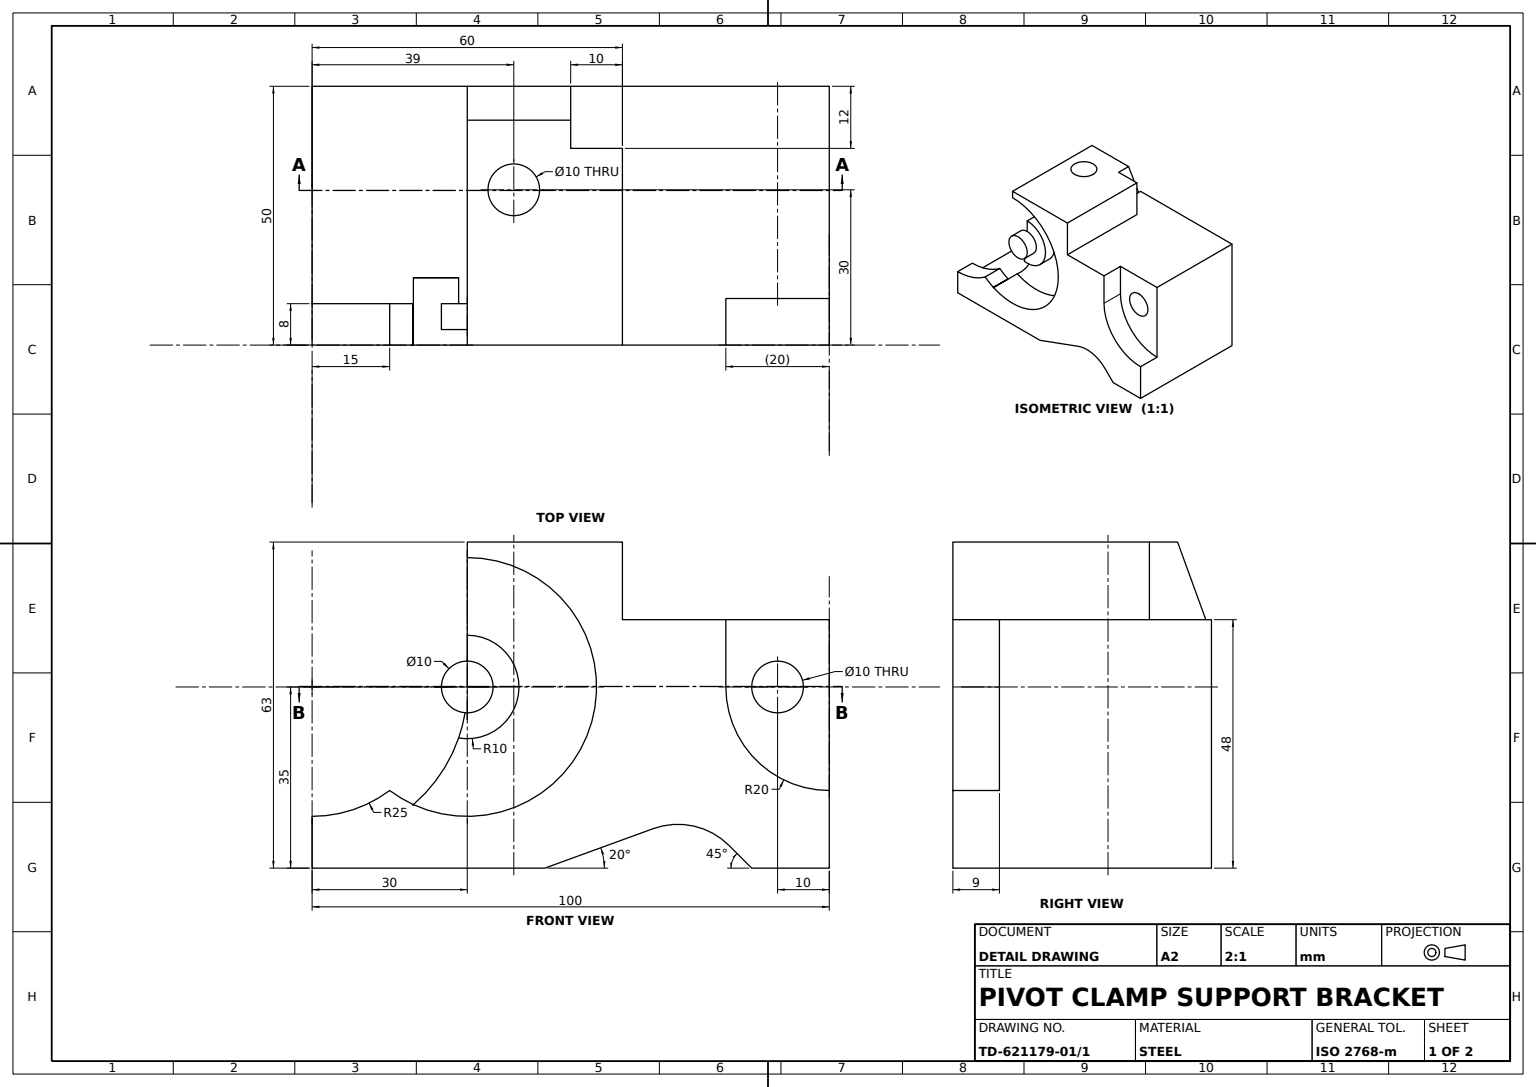
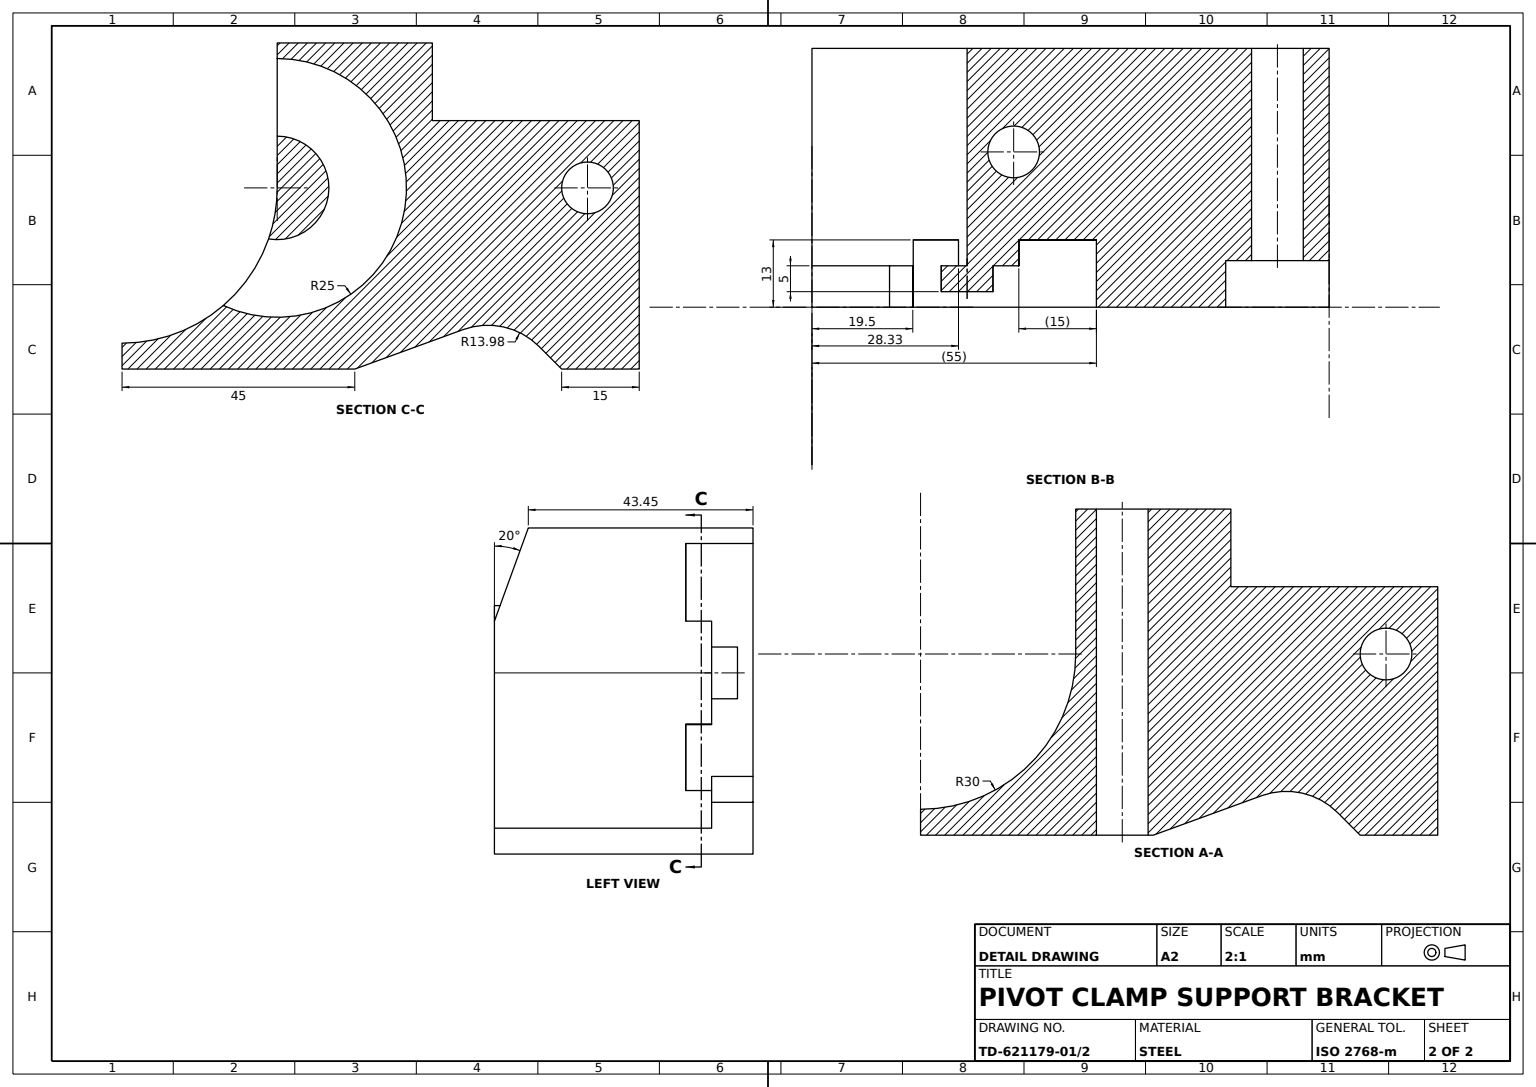
ISO-10303-21;
HEADER;
FILE_DESCRIPTION((''),'2;1');
FILE_NAME('','',(''),(''),'','','');
FILE_SCHEMA(('AUTOMOTIVE_DESIGN'));
ENDSEC;
DATA;
#1=APPLICATION_CONTEXT('');
#2=PRODUCT_CONTEXT('',#1,'mechanical');
#3=PRODUCT('','','',(#2));
#4=PRODUCT_DEFINITION_FORMATION('','',#3);
#5=PRODUCT_DEFINITION_CONTEXT('',#1,'design');
#6=PRODUCT_DEFINITION('','',#4,#5);
#7=PRODUCT_DEFINITION_SHAPE('','',#6);
#8=(LENGTH_UNIT()NAMED_UNIT(*)SI_UNIT(.MILLI.,.METRE.));
#9=(NAMED_UNIT(*)PLANE_ANGLE_UNIT()SI_UNIT($,.RADIAN.));
#10=(NAMED_UNIT(*)SI_UNIT($,.STERADIAN.)SOLID_ANGLE_UNIT());
#11=UNCERTAINTY_MEASURE_WITH_UNIT(LENGTH_MEASURE(0.005),#8,'distance_accuracy_value','');
#12=(GEOMETRIC_REPRESENTATION_CONTEXT(3)GLOBAL_UNCERTAINTY_ASSIGNED_CONTEXT((#11))GLOBAL_UNIT_ASSIGNED_CONTEXT((#8,#9,#10))REPRESENTATION_CONTEXT('',''));
#13=CARTESIAN_POINT('',(-25.,20.954127,-23.873322));
#14=VERTEX_POINT('',#13);
#15=CARTESIAN_POINT('',(25.,20.954127,-23.873322));
#16=VERTEX_POINT('',#15);
#17=CARTESIAN_POINT('',(48.,20.954127,-23.873322));
#18=DIRECTION('',(-1.,0.,0.));
#19=VECTOR('',#18,1000.);
#20=LINE('',#17,#19);
#21=EDGE_CURVE('',#14,#16,#20,.F.);
#22=ORIENTED_EDGE('',*,*,#21,.F.);
#23=CARTESIAN_POINT('',(-25.,35.625997,-27.125997));
#24=VERTEX_POINT('',#23);
#25=CARTESIAN_POINT('',(-25.,25.737223,-37.014771));
#26=DIRECTION('',(1.,0.,0.));
#27=DIRECTION('',(0.,0.,-1.));
#28=AXIS2_PLACEMENT_3D('',#25,#26,#27);
#29=CIRCLE('',#28,13.984838);
#30=EDGE_CURVE('',#24,#14,#29,.T.);
#31=ORIENTED_EDGE('',*,*,#30,.F.);
#32=CARTESIAN_POINT('',(25.,35.625997,-27.125997));
#33=VERTEX_POINT('',#32);
#34=CARTESIAN_POINT('',(48.,35.625997,-27.125997));
#35=LINE('',#34,#19);
#36=EDGE_CURVE('',#24,#33,#35,.F.);
#37=ORIENTED_EDGE('',*,*,#36,.T.);
#38=CARTESIAN_POINT('',(25.,25.737223,-37.014771));
#39=AXIS2_PLACEMENT_3D('',#38,#26,#27);
#40=CIRCLE('',#39,13.984838);
#41=EDGE_CURVE('',#33,#16,#40,.T.);
#42=ORIENTED_EDGE('',*,*,#41,.T.);
#43=EDGE_LOOP('',(#22,#31,#37,#42));
#44=FACE_BOUND('',#43,.T.);
#45=CARTESIAN_POINT('',(48.,25.737223,-37.014771));
#46=DIRECTION('',(0.,0.,1.));
#47=AXIS2_PLACEMENT_3D('',#45,#18,#46);
#48=CYLINDRICAL_SURFACE('',#47,13.984838);
#49=ADVANCED_FACE('',(#44),#48,.F.);
#50=CARTESIAN_POINT('',(17.,-25.5,-19.188103));
#51=VERTEX_POINT('',#50);
#52=CARTESIAN_POINT('',(17.,-30.,-16.5));
#53=VERTEX_POINT('',#52);
#54=CARTESIAN_POINT('',(17.,-15.,3.5));
#55=AXIS2_PLACEMENT_3D('',#54,#26,#27);
#56=CIRCLE('',#55,25.);
#57=EDGE_CURVE('',#51,#53,#56,.F.);
#58=ORIENTED_EDGE('',*,*,#57,.T.);
#59=CARTESIAN_POINT('',(25.,-30.,-16.5));
#60=VERTEX_POINT('',#59);
#61=CARTESIAN_POINT('',(27.5,-30.,-16.5));
#62=LINE('',#61,#19);
#63=EDGE_CURVE('',#60,#53,#62,.T.);
#64=ORIENTED_EDGE('',*,*,#63,.F.);
#65=CARTESIAN_POINT('',(25.,-25.5,-19.188103));
#66=VERTEX_POINT('',#65);
#67=CARTESIAN_POINT('',(25.,-15.,3.5));
#68=AXIS2_PLACEMENT_3D('',#67,#26,#27);
#69=CIRCLE('',#68,25.);
#70=EDGE_CURVE('',#66,#60,#69,.F.);
#71=ORIENTED_EDGE('',*,*,#70,.F.);
#72=CARTESIAN_POINT('',(49.,-25.5,-19.188103));
#73=LINE('',#72,#19);
#74=EDGE_CURVE('',#66,#51,#73,.T.);
#75=ORIENTED_EDGE('',*,*,#74,.T.);
#76=EDGE_LOOP('',(#58,#64,#71,#75));
#77=FACE_BOUND('',#76,.T.);
#78=CARTESIAN_POINT('',(49.,-15.,3.5));
#79=AXIS2_PLACEMENT_3D('',#78,#18,#46);
#80=CYLINDRICAL_SURFACE('',#79,25.);
#81=ADVANCED_FACE('',(#77),#80,.F.);
#82=CARTESIAN_POINT('',(17.,-45.,-21.5));
#83=VERTEX_POINT('',#82);
#84=CARTESIAN_POINT('',(17.,-45.,-26.5));
#85=VERTEX_POINT('',#84);
#86=CARTESIAN_POINT('',(17.,-45.,-16.276455));
#87=VECTOR('',#27,1000.);
#88=LINE('',#86,#87);
#89=EDGE_CURVE('',#83,#85,#88,.T.);
#90=ORIENTED_EDGE('',*,*,#89,.T.);
#91=CARTESIAN_POINT('',(-25.,-45.,-26.5));
#92=VERTEX_POINT('',#91);
#93=CARTESIAN_POINT('',(44.,-45.,-26.5));
#94=LINE('',#93,#19);
#95=EDGE_CURVE('',#92,#85,#94,.F.);
#96=ORIENTED_EDGE('',*,*,#95,.F.);
#97=CARTESIAN_POINT('',(-25.,-45.,-31.5));
#98=VERTEX_POINT('',#97);
#99=CARTESIAN_POINT('',(-25.,-45.,31.5));
#100=LINE('',#99,#87);
#101=EDGE_CURVE('',#92,#98,#100,.T.);
#102=ORIENTED_EDGE('',*,*,#101,.T.);
#103=CARTESIAN_POINT('',(25.,-45.,-31.5));
#104=VERTEX_POINT('',#103);
#105=LINE('',#103,#19);
#106=EDGE_CURVE('',#104,#98,#105,.T.);
#107=ORIENTED_EDGE('',*,*,#106,.F.);
#108=CARTESIAN_POINT('',(25.,-45.,-21.5));
#109=VERTEX_POINT('',#108);
#110=CARTESIAN_POINT('',(25.,-45.,31.5));
#111=LINE('',#110,#87);
#112=EDGE_CURVE('',#109,#104,#111,.T.);
#113=ORIENTED_EDGE('',*,*,#112,.F.);
#114=CARTESIAN_POINT('',(28.,-45.,-21.5));
#115=LINE('',#114,#19);
#116=EDGE_CURVE('',#83,#109,#115,.F.);
#117=ORIENTED_EDGE('',*,*,#116,.F.);
#118=EDGE_LOOP('',(#90,#96,#102,#107,#113,#117));
#119=FACE_BOUND('',#118,.T.);
#120=DIRECTION('',(0.,1.,0.));
#121=AXIS2_PLACEMENT_3D('',#110,#120,#46);
#122=PLANE('',#121);
#123=ADVANCED_FACE('',(#119),#122,.F.);
#124=CARTESIAN_POINT('',(22.,-10.,3.5));
#125=VERTEX_POINT('',#124);
#126=CARTESIAN_POINT('',(22.,-15.,3.5));
#127=AXIS2_PLACEMENT_3D('',#126,#26,#120);
#128=CIRCLE('',#127,5.);
#129=EDGE_CURVE('',#125,#125,#128,.T.);
#130=ORIENTED_EDGE('',*,*,#129,.T.);
#131=EDGE_LOOP('',(#130));
#132=FACE_BOUND('',#131,.T.);
#133=AXIS2_PLACEMENT_3D('',#126,#26,#27);
#134=PLANE('',#133);
#135=ADVANCED_FACE('',(#132),#134,.T.);
#136=CARTESIAN_POINT('',(-23.908089,5.,16.5));
#137=VERTEX_POINT('',#136);
#138=CARTESIAN_POINT('',(-18.448536,5.,31.5));
#139=VERTEX_POINT('',#138);
#140=CARTESIAN_POINT('',(-25.,5.,13.5));
#141=DIRECTION('',(0.342020143,0.,0.939692621));
#142=VECTOR('',#141,1000.);
#143=LINE('',#140,#142);
#144=EDGE_CURVE('',#137,#139,#143,.T.);
#145=ORIENTED_EDGE('',*,*,#144,.T.);
#146=CARTESIAN_POINT('',(-13.,5.,31.5));
#147=VERTEX_POINT('',#146);
#148=CARTESIAN_POINT('',(25.,5.,31.5));
#149=VECTOR('',#26,1000.);
#150=LINE('',#148,#149);
#151=EDGE_CURVE('',#139,#147,#150,.T.);
#152=ORIENTED_EDGE('',*,*,#151,.T.);
#153=CARTESIAN_POINT('',(-13.,5.,16.5));
#154=VERTEX_POINT('',#153);
#155=CARTESIAN_POINT('',(-13.,5.,48.));
#156=LINE('',#155,#87);
#157=EDGE_CURVE('',#154,#147,#156,.F.);
#158=ORIENTED_EDGE('',*,*,#157,.F.);
#159=CARTESIAN_POINT('',(-25.,5.,16.5));
#160=LINE('',#159,#149);
#161=EDGE_CURVE('',#137,#154,#160,.T.);
#162=ORIENTED_EDGE('',*,*,#161,.F.);
#163=EDGE_LOOP('',(#145,#152,#158,#162));
#164=FACE_BOUND('',#163,.T.);
#165=CARTESIAN_POINT('',(-25.,5.,48.));
#166=AXIS2_PLACEMENT_3D('',#165,#120,#18);
#167=PLANE('',#166);
#168=ADVANCED_FACE('',(#164),#167,.T.);
#169=CARTESIAN_POINT('',(-5.,-1.,31.5));
#170=VERTEX_POINT('',#169);
#171=CARTESIAN_POINT('',(-5.,-6.,31.5));
#172=AXIS2_PLACEMENT_3D('',#171,#27,#120);
#173=CIRCLE('',#172,5.);
#174=EDGE_CURVE('',#170,#170,#173,.T.);
#175=ORIENTED_EDGE('',*,*,#174,.F.);
#176=EDGE_LOOP('',(#175));
#177=FACE_BOUND('',#176,.T.);
#178=CARTESIAN_POINT('',(-5.,-11.,-31.5));
#179=VERTEX_POINT('',#178);
#180=CARTESIAN_POINT('',(-5.,-6.,-31.5));
#181=DIRECTION('',(0.,-1.,0.));
#182=AXIS2_PLACEMENT_3D('',#180,#46,#181);
#183=CIRCLE('',#182,5.);
#184=EDGE_CURVE('',#179,#179,#183,.T.);
#185=ORIENTED_EDGE('',*,*,#184,.F.);
#186=EDGE_LOOP('',(#185));
#187=FACE_BOUND('',#186,.T.);
#188=CYLINDRICAL_SURFACE('',#172,5.);
#189=ADVANCED_FACE('',(#177,#187),#188,.F.);
#190=CARTESIAN_POINT('',(25.,-15.,31.5));
#191=VERTEX_POINT('',#190);
#192=CARTESIAN_POINT('',(25.,-15.,28.5));
#193=VERTEX_POINT('',#192);
#194=CARTESIAN_POINT('',(25.,-15.,0.));
#195=LINE('',#194,#87);
#196=EDGE_CURVE('',#191,#193,#195,.T.);
#197=ORIENTED_EDGE('',*,*,#196,.F.);
#198=CARTESIAN_POINT('',(-18.448536,-15.,31.5));
#199=VERTEX_POINT('',#198);
#200=LINE('',#190,#19);
#201=EDGE_CURVE('',#191,#199,#200,.T.);
#202=ORIENTED_EDGE('',*,*,#201,.T.);
#203=CARTESIAN_POINT('',(-25.,-15.,13.5));
#204=VERTEX_POINT('',#203);
#205=CARTESIAN_POINT('',(-20.142471,-15.,26.84595));
#206=DIRECTION('',(-0.342020143,0.,-0.939692621));
#207=VECTOR('',#206,1000.);
#208=LINE('',#205,#207);
#209=EDGE_CURVE('',#199,#204,#208,.T.);
#210=ORIENTED_EDGE('',*,*,#209,.T.);
#211=CARTESIAN_POINT('',(-25.,-15.,3.5));
#212=VERTEX_POINT('',#211);
#213=CARTESIAN_POINT('',(-25.,-15.,0.));
#214=LINE('',#213,#87);
#215=EDGE_CURVE('',#204,#212,#214,.T.);
#216=ORIENTED_EDGE('',*,*,#215,.T.);
#217=VERTEX_POINT('',#54);
#218=CARTESIAN_POINT('',(44.,-15.,3.5));
#219=LINE('',#218,#19);
#220=EDGE_CURVE('',#212,#217,#219,.F.);
#221=ORIENTED_EDGE('',*,*,#220,.T.);
#222=CARTESIAN_POINT('',(17.,-15.,8.5));
#223=VERTEX_POINT('',#222);
#224=LINE('',#54,#87);
#225=EDGE_CURVE('',#223,#217,#224,.T.);
#226=ORIENTED_EDGE('',*,*,#225,.F.);
#227=CARTESIAN_POINT('',(17.,-15.,13.5));
#228=VERTEX_POINT('',#227);
#229=EDGE_CURVE('',#228,#223,#224,.T.);
#230=ORIENTED_EDGE('',*,*,#229,.F.);
#231=CARTESIAN_POINT('',(12.,-15.,13.5));
#232=VERTEX_POINT('',#231);
#233=LINE('',#227,#19);
#234=EDGE_CURVE('',#228,#232,#233,.T.);
#235=ORIENTED_EDGE('',*,*,#234,.T.);
#236=CARTESIAN_POINT('',(12.,-15.,28.5));
#237=VERTEX_POINT('',#236);
#238=CARTESIAN_POINT('',(12.,-15.,3.5));
#239=VECTOR('',#46,1000.);
#240=LINE('',#238,#239);
#241=EDGE_CURVE('',#232,#237,#240,.T.);
#242=ORIENTED_EDGE('',*,*,#241,.T.);
#243=CARTESIAN_POINT('',(30.,-15.,28.5));
#244=LINE('',#243,#19);
#245=EDGE_CURVE('',#237,#193,#244,.F.);
#246=ORIENTED_EDGE('',*,*,#245,.T.);
#247=EDGE_LOOP('',(#197,#202,#210,#216,#221,#226,#230,#235,#242,#246));
#248=FACE_BOUND('',#247,.T.);
#249=AXIS2_PLACEMENT_3D('',#218,#181,#27);
#250=PLANE('',#249);
#251=ADVANCED_FACE('',(#248),#250,.T.);
#252=CARTESIAN_POINT('',(-13.,15.,31.5));
#253=VERTEX_POINT('',#252);
#254=CARTESIAN_POINT('',(-13.,55.,31.5));
#255=VECTOR('',#120,1000.);
#256=LINE('',#254,#255);
#257=EDGE_CURVE('',#147,#253,#256,.T.);
#258=ORIENTED_EDGE('',*,*,#257,.T.);
#259=CARTESIAN_POINT('',(-13.,15.,16.5));
#260=VERTEX_POINT('',#259);
#261=CARTESIAN_POINT('',(-13.,15.,48.));
#262=LINE('',#261,#87);
#263=EDGE_CURVE('',#253,#260,#262,.T.);
#264=ORIENTED_EDGE('',*,*,#263,.T.);
#265=LINE('',#153,#255);
#266=EDGE_CURVE('',#154,#260,#265,.T.);
#267=ORIENTED_EDGE('',*,*,#266,.F.);
#268=ORIENTED_EDGE('',*,*,#157,.T.);
#269=EDGE_LOOP('',(#258,#264,#267,#268));
#270=FACE_BOUND('',#269,.T.);
#271=AXIS2_PLACEMENT_3D('',#155,#18,#181);
#272=PLANE('',#271);
#273=ADVANCED_FACE('',(#270),#272,.T.);
#274=CARTESIAN_POINT('',(-25.,40.,-31.5));
#275=VERTEX_POINT('',#274);
#276=CARTESIAN_POINT('',(-25.,4.25,4.25));
#277=DIRECTION('',(0.,-0.707106781,0.707106781));
#278=VECTOR('',#277,1000.);
#279=LINE('',#276,#278);
#280=EDGE_CURVE('',#275,#24,#279,.T.);
#281=ORIENTED_EDGE('',*,*,#280,.F.);
#282=CARTESIAN_POINT('',(25.,40.,-31.5));
#283=VERTEX_POINT('',#282);
#284=CARTESIAN_POINT('',(48.,40.,-31.5));
#285=LINE('',#284,#19);
#286=EDGE_CURVE('',#283,#275,#285,.T.);
#287=ORIENTED_EDGE('',*,*,#286,.F.);
#288=CARTESIAN_POINT('',(25.,4.25,4.25));
#289=LINE('',#288,#278);
#290=EDGE_CURVE('',#283,#33,#289,.T.);
#291=ORIENTED_EDGE('',*,*,#290,.T.);
#292=ORIENTED_EDGE('',*,*,#36,.F.);
#293=EDGE_LOOP('',(#281,#287,#291,#292));
#294=FACE_BOUND('',#293,.T.);
#295=DIRECTION('',(0.,0.707106781,0.707106781));
#296=AXIS2_PLACEMENT_3D('',#34,#295,#277);
#297=PLANE('',#296);
#298=ADVANCED_FACE('',(#294),#297,.F.);
#299=CARTESIAN_POINT('',(16.,45.,8.5));
#300=VERTEX_POINT('',#299);
#301=CARTESIAN_POINT('',(16.,45.,3.5));
#302=AXIS2_PLACEMENT_3D('',#301,#18,#46);
#303=CIRCLE('',#302,5.);
#304=EDGE_CURVE('',#300,#300,#303,.T.);
#305=ORIENTED_EDGE('',*,*,#304,.F.);
#306=EDGE_LOOP('',(#305));
#307=FACE_BOUND('',#306,.T.);
#308=CARTESIAN_POINT('',(-25.,45.,-1.5));
#309=VERTEX_POINT('',#308);
#310=CARTESIAN_POINT('',(-25.,45.,3.5));
#311=AXIS2_PLACEMENT_3D('',#310,#26,#27);
#312=CIRCLE('',#311,5.);
#313=EDGE_CURVE('',#309,#309,#312,.T.);
#314=ORIENTED_EDGE('',*,*,#313,.F.);
#315=EDGE_LOOP('',(#314));
#316=FACE_BOUND('',#315,.T.);
#317=CYLINDRICAL_SURFACE('',#302,5.);
#318=ADVANCED_FACE('',(#307,#316),#317,.F.);
#319=ORIENTED_EDGE('',*,*,#304,.T.);
#320=EDGE_LOOP('',(#319));
#321=FACE_BOUND('',#320,.T.);
#322=CARTESIAN_POINT('',(16.,55.,-16.5));
#323=VERTEX_POINT('',#322);
#324=CARTESIAN_POINT('',(16.,55.,16.5));
#325=VERTEX_POINT('',#324);
#326=LINE('',#322,#239);
#327=EDGE_CURVE('',#323,#325,#326,.T.);
#328=ORIENTED_EDGE('',*,*,#327,.T.);
#329=CARTESIAN_POINT('',(16.,35.,16.5));
#330=VERTEX_POINT('',#329);
#331=LINE('',#324,#255);
#332=EDGE_CURVE('',#330,#325,#331,.T.);
#333=ORIENTED_EDGE('',*,*,#332,.F.);
#334=CARTESIAN_POINT('',(16.,35.,3.5));
#335=VERTEX_POINT('',#334);
#336=CARTESIAN_POINT('',(16.,35.,20.));
#337=LINE('',#336,#87);
#338=EDGE_CURVE('',#335,#330,#337,.F.);
#339=ORIENTED_EDGE('',*,*,#338,.F.);
#340=CARTESIAN_POINT('',(16.,55.,3.5));
#341=AXIS2_PLACEMENT_3D('',#340,#26,#120);
#342=CIRCLE('',#341,20.);
#343=EDGE_CURVE('',#323,#335,#342,.F.);
#344=ORIENTED_EDGE('',*,*,#343,.F.);
#345=EDGE_LOOP('',(#328,#333,#339,#344));
#346=FACE_BOUND('',#345,.T.);
#347=AXIS2_PLACEMENT_3D('',#340,#26,#27);
#348=PLANE('',#347);
#349=ADVANCED_FACE('',(#321,#346),#348,.T.);
#350=VERTEX_POINT('',#140);
#351=EDGE_CURVE('',#137,#350,#143,.F.);
#352=ORIENTED_EDGE('',*,*,#351,.T.);
#353=CARTESIAN_POINT('',(-25.,-25.,13.5));
#354=LINE('',#353,#255);
#355=EDGE_CURVE('',#204,#350,#354,.T.);
#356=ORIENTED_EDGE('',*,*,#355,.F.);
#357=ORIENTED_EDGE('',*,*,#209,.F.);
#358=CARTESIAN_POINT('',(-18.448536,-25.,31.5));
#359=LINE('',#358,#255);
#360=EDGE_CURVE('',#199,#139,#359,.T.);
#361=ORIENTED_EDGE('',*,*,#360,.T.);
#362=ORIENTED_EDGE('',*,*,#144,.F.);
#363=EDGE_LOOP('',(#352,#356,#357,#361,#362));
#364=FACE_BOUND('',#363,.T.);
#365=DIRECTION('',(-0.939692621,0.,0.342020143));
#366=AXIS2_PLACEMENT_3D('',#353,#365,#141);
#367=PLANE('',#366);
#368=ADVANCED_FACE('',(#364),#367,.T.);
#369=CARTESIAN_POINT('',(12.,-16.666667,-6.360133));
#370=VERTEX_POINT('',#369);
#371=CARTESIAN_POINT('',(17.,-16.666667,-6.360133));
#372=VERTEX_POINT('',#371);
#373=CARTESIAN_POINT('',(0.,-16.666667,-6.360133));
#374=LINE('',#373,#19);
#375=EDGE_CURVE('',#370,#372,#374,.F.);
#376=ORIENTED_EDGE('',*,*,#375,.T.);
#377=CARTESIAN_POINT('',(17.,-15.416667,-1.482609));
#378=VERTEX_POINT('',#377);
#379=CARTESIAN_POINT('',(17.,-45.,3.5));
#380=AXIS2_PLACEMENT_3D('',#379,#26,#27);
#381=CIRCLE('',#380,30.);
#382=EDGE_CURVE('',#378,#372,#381,.F.);
#383=ORIENTED_EDGE('',*,*,#382,.F.);
#384=EDGE_CURVE('',#217,#378,#381,.F.);
#385=ORIENTED_EDGE('',*,*,#384,.F.);
#386=ORIENTED_EDGE('',*,*,#220,.F.);
#387=CARTESIAN_POINT('',(-25.,-45.,3.5));
#388=AXIS2_PLACEMENT_3D('',#387,#26,#27);
#389=CIRCLE('',#388,30.);
#390=EDGE_CURVE('',#212,#92,#389,.F.);
#391=ORIENTED_EDGE('',*,*,#390,.T.);
#392=ORIENTED_EDGE('',*,*,#95,.T.);
#393=CARTESIAN_POINT('',(17.,-25.5,-19.298026));
#394=VERTEX_POINT('',#393);
#395=EDGE_CURVE('',#85,#394,#381,.T.);
#396=ORIENTED_EDGE('',*,*,#395,.T.);
#397=CARTESIAN_POINT('',(25.,-25.5,-19.298026));
#398=VERTEX_POINT('',#397);
#399=CARTESIAN_POINT('',(44.,-25.5,-19.298026));
#400=LINE('',#399,#19);
#401=EDGE_CURVE('',#394,#398,#400,.F.);
#402=ORIENTED_EDGE('',*,*,#401,.T.);
#403=CARTESIAN_POINT('',(25.,-25.416667,-19.226484));
#404=VERTEX_POINT('',#403);
#405=CARTESIAN_POINT('',(25.,-45.,3.5));
#406=AXIS2_PLACEMENT_3D('',#405,#26,#27);
#407=CIRCLE('',#406,30.);
#408=EDGE_CURVE('',#404,#398,#407,.F.);
#409=ORIENTED_EDGE('',*,*,#408,.F.);
#410=CARTESIAN_POINT('',(12.,-25.416667,-19.226484));
#411=VERTEX_POINT('',#410);
#412=CARTESIAN_POINT('',(0.,-25.416667,-19.226484));
#413=LINE('',#412,#19);
#414=EDGE_CURVE('',#404,#411,#413,.T.);
#415=ORIENTED_EDGE('',*,*,#414,.T.);
#416=CARTESIAN_POINT('',(12.,-45.,3.5));
#417=AXIS2_PLACEMENT_3D('',#416,#18,#46);
#418=CIRCLE('',#417,30.);
#419=EDGE_CURVE('',#411,#370,#418,.F.);
#420=ORIENTED_EDGE('',*,*,#419,.T.);
#421=EDGE_LOOP('',(#376,#383,#385,#386,#391,#392,#396,#402,#409,#415,#420));
#422=FACE_BOUND('',#421,.T.);
#423=CARTESIAN_POINT('',(44.,-45.,3.5));
#424=AXIS2_PLACEMENT_3D('',#423,#18,#46);
#425=CYLINDRICAL_SURFACE('',#424,30.);
#426=ADVANCED_FACE('',(#422),#425,.F.);
#427=ORIENTED_EDGE('',*,*,#390,.F.);
#428=ORIENTED_EDGE('',*,*,#215,.F.);
#429=ORIENTED_EDGE('',*,*,#355,.T.);
#430=VERTEX_POINT('',#159);
#431=CARTESIAN_POINT('',(-25.,5.,31.5));
#432=LINE('',#431,#87);
#433=EDGE_CURVE('',#430,#350,#432,.T.);
#434=ORIENTED_EDGE('',*,*,#433,.F.);
#435=CARTESIAN_POINT('',(-25.,55.,16.5));
#436=VERTEX_POINT('',#435);
#437=CARTESIAN_POINT('',(-25.,0.,16.5));
#438=LINE('',#437,#255);
#439=EDGE_CURVE('',#430,#436,#438,.T.);
#440=ORIENTED_EDGE('',*,*,#439,.T.);
#441=CARTESIAN_POINT('',(-25.,55.,-31.5));
#442=VERTEX_POINT('',#441);
#443=LINE('',#441,#239);
#444=EDGE_CURVE('',#442,#436,#443,.T.);
#445=ORIENTED_EDGE('',*,*,#444,.F.);
#446=LINE('',#97,#255);
#447=EDGE_CURVE('',#275,#442,#446,.T.);
#448=ORIENTED_EDGE('',*,*,#447,.F.);
#449=ORIENTED_EDGE('',*,*,#280,.T.);
#450=ORIENTED_EDGE('',*,*,#30,.T.);
#451=CARTESIAN_POINT('',(-25.,0.,-31.5));
#452=VERTEX_POINT('',#451);
#453=CARTESIAN_POINT('',(-25.,10.123905,-27.8152));
#454=DIRECTION('',(0.,-0.939692621,-0.342020143));
#455=VECTOR('',#454,1000.);
#456=LINE('',#453,#455);
#457=EDGE_CURVE('',#14,#452,#456,.T.);
#458=ORIENTED_EDGE('',*,*,#457,.T.);
#459=EDGE_CURVE('',#98,#452,#446,.T.);
#460=ORIENTED_EDGE('',*,*,#459,.F.);
#461=ORIENTED_EDGE('',*,*,#101,.F.);
#462=EDGE_LOOP('',(#427,#428,#429,#434,#440,#445,#448,#449,#450,#458,#460,#461));
#463=FACE_BOUND('',#462,.T.);
#464=ORIENTED_EDGE('',*,*,#313,.T.);
#465=EDGE_LOOP('',(#464));
#466=FACE_BOUND('',#465,.T.);
#467=CARTESIAN_POINT('',(-25.,0.,0.));
#468=AXIS2_PLACEMENT_3D('',#467,#26,#27);
#469=PLANE('',#468);
#470=ADVANCED_FACE('',(#463,#466),#469,.F.);
#471=ORIENTED_EDGE('',*,*,#375,.F.);
#472=AXIS2_PLACEMENT_3D('',#238,#18,#46);
#473=CIRCLE('',#472,10.);
#474=EDGE_CURVE('',#370,#232,#473,.F.);
#475=ORIENTED_EDGE('',*,*,#474,.T.);
#476=ORIENTED_EDGE('',*,*,#234,.F.);
#477=AXIS2_PLACEMENT_3D('',#54,#26,#120);
#478=CIRCLE('',#477,10.);
#479=EDGE_CURVE('',#372,#228,#478,.T.);
#480=ORIENTED_EDGE('',*,*,#479,.F.);
#481=EDGE_LOOP('',(#471,#475,#476,#480));
#482=FACE_BOUND('',#481,.T.);
#483=AXIS2_PLACEMENT_3D('',#54,#18,#46);
#484=CYLINDRICAL_SURFACE('',#483,10.);
#485=ADVANCED_FACE('',(#482),#484,.T.);
#486=ORIENTED_EDGE('',*,*,#433,.T.);
#487=ORIENTED_EDGE('',*,*,#351,.F.);
#488=EDGE_CURVE('',#137,#430,#160,.F.);
#489=ORIENTED_EDGE('',*,*,#488,.T.);
#490=EDGE_LOOP('',(#486,#487,#489));
#491=FACE_BOUND('',#490,.T.);
#492=CARTESIAN_POINT('',(0.,5.,0.));
#493=AXIS2_PLACEMENT_3D('',#492,#181,#27);
#494=PLANE('',#493);
#495=ADVANCED_FACE('',(#491),#494,.T.);
#496=ORIENTED_EDGE('',*,*,#106,.T.);
#497=ORIENTED_EDGE('',*,*,#459,.T.);
#498=CARTESIAN_POINT('',(25.,0.,-31.5));
#499=VERTEX_POINT('',#498);
#500=CARTESIAN_POINT('',(48.,0.,-31.5));
#501=LINE('',#500,#19);
#502=EDGE_CURVE('',#499,#452,#501,.T.);
#503=ORIENTED_EDGE('',*,*,#502,.F.);
#504=LINE('',#103,#255);
#505=EDGE_CURVE('',#104,#499,#504,.T.);
#506=ORIENTED_EDGE('',*,*,#505,.F.);
#507=EDGE_LOOP('',(#496,#497,#503,#506));
#508=FACE_BOUND('',#507,.T.);
#509=ORIENTED_EDGE('',*,*,#184,.T.);
#510=EDGE_LOOP('',(#509));
#511=FACE_BOUND('',#510,.T.);
#512=AXIS2_PLACEMENT_3D('',#103,#46,#181);
#513=PLANE('',#512);
#514=ADVANCED_FACE('',(#508,#511),#513,.F.);
#515=ORIENTED_EDGE('',*,*,#263,.F.);
#516=CARTESIAN_POINT('',(25.,15.,31.5));
#517=VERTEX_POINT('',#516);
#518=LINE('',#516,#19);
#519=EDGE_CURVE('',#517,#253,#518,.T.);
#520=ORIENTED_EDGE('',*,*,#519,.F.);
#521=CARTESIAN_POINT('',(25.,15.,16.5));
#522=VERTEX_POINT('',#521);
#523=CARTESIAN_POINT('',(25.,15.,0.));
#524=LINE('',#523,#87);
#525=EDGE_CURVE('',#517,#522,#524,.T.);
#526=ORIENTED_EDGE('',*,*,#525,.T.);
#527=CARTESIAN_POINT('',(30.,15.,16.5));
#528=LINE('',#527,#19);
#529=EDGE_CURVE('',#260,#522,#528,.F.);
#530=ORIENTED_EDGE('',*,*,#529,.F.);
#531=EDGE_LOOP('',(#515,#520,#526,#530));
#532=FACE_BOUND('',#531,.T.);
#533=CARTESIAN_POINT('',(30.,15.,48.));
#534=AXIS2_PLACEMENT_3D('',#533,#181,#27);
#535=PLANE('',#534);
#536=ADVANCED_FACE('',(#532),#535,.F.);
#537=CIRCLE('',#477,5.);
#538=EDGE_CURVE('',#378,#223,#537,.T.);
#539=ORIENTED_EDGE('',*,*,#538,.T.);
#540=EDGE_CURVE('',#223,#378,#537,.T.);
#541=ORIENTED_EDGE('',*,*,#540,.T.);
#542=EDGE_LOOP('',(#539,#541));
#543=FACE_BOUND('',#542,.T.);
#544=ORIENTED_EDGE('',*,*,#129,.F.);
#545=EDGE_LOOP('',(#544));
#546=FACE_BOUND('',#545,.T.);
#547=AXIS2_PLACEMENT_3D('',#126,#18,#46);
#548=CYLINDRICAL_SURFACE('',#547,5.);
#549=ADVANCED_FACE('',(#543,#546),#548,.T.);
#550=ORIENTED_EDGE('',*,*,#338,.T.);
#551=CARTESIAN_POINT('',(25.,35.,16.5));
#552=VERTEX_POINT('',#551);
#553=CARTESIAN_POINT('',(39.,35.,16.5));
#554=LINE('',#553,#19);
#555=EDGE_CURVE('',#330,#552,#554,.F.);
#556=ORIENTED_EDGE('',*,*,#555,.T.);
#557=CARTESIAN_POINT('',(25.,35.,3.5));
#558=VERTEX_POINT('',#557);
#559=CARTESIAN_POINT('',(25.,35.,0.));
#560=LINE('',#559,#239);
#561=EDGE_CURVE('',#558,#552,#560,.T.);
#562=ORIENTED_EDGE('',*,*,#561,.F.);
#563=CARTESIAN_POINT('',(39.,35.,3.5));
#564=LINE('',#563,#19);
#565=EDGE_CURVE('',#335,#558,#564,.F.);
#566=ORIENTED_EDGE('',*,*,#565,.F.);
#567=EDGE_LOOP('',(#550,#556,#562,#566));
#568=FACE_BOUND('',#567,.T.);
#569=CARTESIAN_POINT('',(39.,35.,20.));
#570=AXIS2_PLACEMENT_3D('',#569,#120,#46);
#571=PLANE('',#570);
#572=ADVANCED_FACE('',(#568),#571,.T.);
#573=ORIENTED_EDGE('',*,*,#241,.F.);
#574=ORIENTED_EDGE('',*,*,#474,.F.);
#575=ORIENTED_EDGE('',*,*,#419,.F.);
#576=CIRCLE('',#472,25.);
#577=EDGE_CURVE('',#411,#237,#576,.F.);
#578=ORIENTED_EDGE('',*,*,#577,.T.);
#579=EDGE_LOOP('',(#573,#574,#575,#578));
#580=FACE_BOUND('',#579,.T.);
#581=PLANE('',#472);
#582=ADVANCED_FACE('',(#580),#581,.F.);
#583=ORIENTED_EDGE('',*,*,#245,.F.);
#584=ORIENTED_EDGE('',*,*,#577,.F.);
#585=ORIENTED_EDGE('',*,*,#414,.F.);
#586=EDGE_CURVE('',#404,#193,#69,.T.);
#587=ORIENTED_EDGE('',*,*,#586,.T.);
#588=EDGE_LOOP('',(#583,#584,#585,#587));
#589=FACE_BOUND('',#588,.T.);
#590=CARTESIAN_POINT('',(30.,-15.,3.5));
#591=AXIS2_PLACEMENT_3D('',#590,#18,#46);
#592=CYLINDRICAL_SURFACE('',#591,25.);
#593=ADVANCED_FACE('',(#589),#592,.F.);
#594=ORIENTED_EDGE('',*,*,#229,.T.);
#595=ORIENTED_EDGE('',*,*,#538,.F.);
#596=ORIENTED_EDGE('',*,*,#382,.T.);
#597=ORIENTED_EDGE('',*,*,#479,.T.);
#598=EDGE_LOOP('',(#594,#595,#596,#597));
#599=FACE_BOUND('',#598,.T.);
#600=PLANE('',#55);
#601=ADVANCED_FACE('',(#599),#600,.T.);
#602=CARTESIAN_POINT('',(25.,-25.5,-31.5));
#603=LINE('',#602,#239);
#604=EDGE_CURVE('',#398,#66,#603,.T.);
#605=ORIENTED_EDGE('',*,*,#604,.T.);
#606=ORIENTED_EDGE('',*,*,#70,.T.);
#607=CIRCLE('',#406,25.);
#608=EDGE_CURVE('',#60,#109,#607,.F.);
#609=ORIENTED_EDGE('',*,*,#608,.T.);
#610=ORIENTED_EDGE('',*,*,#112,.T.);
#611=ORIENTED_EDGE('',*,*,#505,.T.);
#612=CARTESIAN_POINT('',(25.,10.123905,-27.8152));
#613=LINE('',#612,#455);
#614=EDGE_CURVE('',#16,#499,#613,.T.);
#615=ORIENTED_EDGE('',*,*,#614,.F.);
#616=ORIENTED_EDGE('',*,*,#41,.F.);
#617=ORIENTED_EDGE('',*,*,#290,.F.);
#618=CARTESIAN_POINT('',(25.,55.,-31.5));
#619=VERTEX_POINT('',#618);
#620=EDGE_CURVE('',#283,#619,#504,.T.);
#621=ORIENTED_EDGE('',*,*,#620,.T.);
#622=CARTESIAN_POINT('',(25.,55.,-16.5));
#623=VERTEX_POINT('',#622);
#624=LINE('',#618,#239);
#625=EDGE_CURVE('',#619,#623,#624,.T.);
#626=ORIENTED_EDGE('',*,*,#625,.T.);
#627=CARTESIAN_POINT('',(25.,55.,3.5));
#628=AXIS2_PLACEMENT_3D('',#627,#26,#27);
#629=CIRCLE('',#628,20.);
#630=EDGE_CURVE('',#623,#558,#629,.F.);
#631=ORIENTED_EDGE('',*,*,#630,.T.);
#632=ORIENTED_EDGE('',*,*,#561,.T.);
#633=CARTESIAN_POINT('',(25.,0.,16.5));
#634=LINE('',#633,#255);
#635=EDGE_CURVE('',#522,#552,#634,.T.);
#636=ORIENTED_EDGE('',*,*,#635,.F.);
#637=ORIENTED_EDGE('',*,*,#525,.F.);
#638=CARTESIAN_POINT('',(25.,55.,31.5));
#639=VECTOR('',#181,1000.);
#640=LINE('',#638,#639);
#641=EDGE_CURVE('',#517,#191,#640,.T.);
#642=ORIENTED_EDGE('',*,*,#641,.T.);
#643=ORIENTED_EDGE('',*,*,#196,.T.);
#644=ORIENTED_EDGE('',*,*,#586,.F.);
#645=ORIENTED_EDGE('',*,*,#408,.T.);
#646=EDGE_LOOP('',(#605,#606,#609,#610,#611,#615,#616,#617,#621,#626,#631,#632,#636,#637,#642,#643,#644,#645));
#647=FACE_BOUND('',#646,.T.);
#648=CARTESIAN_POINT('',(25.,0.,0.));
#649=AXIS2_PLACEMENT_3D('',#648,#26,#27);
#650=PLANE('',#649);
#651=ADVANCED_FACE('',(#647),#650,.T.);
#652=ORIENTED_EDGE('',*,*,#332,.T.);
#653=CARTESIAN_POINT('',(-30.,55.,16.5));
#654=LINE('',#653,#149);
#655=EDGE_CURVE('',#436,#325,#654,.T.);
#656=ORIENTED_EDGE('',*,*,#655,.F.);
#657=ORIENTED_EDGE('',*,*,#439,.F.);
#658=ORIENTED_EDGE('',*,*,#488,.F.);
#659=ORIENTED_EDGE('',*,*,#161,.T.);
#660=ORIENTED_EDGE('',*,*,#266,.T.);
#661=ORIENTED_EDGE('',*,*,#529,.T.);
#662=ORIENTED_EDGE('',*,*,#635,.T.);
#663=ORIENTED_EDGE('',*,*,#555,.F.);
#664=EDGE_LOOP('',(#652,#656,#657,#658,#659,#660,#661,#662,#663));
#665=FACE_BOUND('',#664,.T.);
#666=CARTESIAN_POINT('',(0.,0.,16.5));
#667=AXIS2_PLACEMENT_3D('',#666,#27,#18);
#668=PLANE('',#667);
#669=ADVANCED_FACE('',(#665),#668,.F.);
#670=ORIENTED_EDGE('',*,*,#565,.T.);
#671=ORIENTED_EDGE('',*,*,#630,.F.);
#672=CARTESIAN_POINT('',(39.,55.,-16.5));
#673=LINE('',#672,#19);
#674=EDGE_CURVE('',#623,#323,#673,.T.);
#675=ORIENTED_EDGE('',*,*,#674,.T.);
#676=ORIENTED_EDGE('',*,*,#343,.T.);
#677=EDGE_LOOP('',(#670,#671,#675,#676));
#678=FACE_BOUND('',#677,.T.);
#679=CARTESIAN_POINT('',(39.,55.,3.5));
#680=AXIS2_PLACEMENT_3D('',#679,#18,#46);
#681=CYLINDRICAL_SURFACE('',#680,20.);
#682=ADVANCED_FACE('',(#678),#681,.F.);
#683=ORIENTED_EDGE('',*,*,#384,.T.);
#684=ORIENTED_EDGE('',*,*,#540,.F.);
#685=ORIENTED_EDGE('',*,*,#225,.T.);
#686=EDGE_LOOP('',(#683,#684,#685));
#687=FACE_BOUND('',#686,.T.);
#688=ADVANCED_FACE('',(#687),#600,.F.);
#689=ORIENTED_EDGE('',*,*,#174,.T.);
#690=EDGE_LOOP('',(#689));
#691=FACE_BOUND('',#690,.T.);
#692=ORIENTED_EDGE('',*,*,#360,.F.);
#693=ORIENTED_EDGE('',*,*,#201,.F.);
#694=ORIENTED_EDGE('',*,*,#641,.F.);
#695=ORIENTED_EDGE('',*,*,#519,.T.);
#696=ORIENTED_EDGE('',*,*,#257,.F.);
#697=ORIENTED_EDGE('',*,*,#151,.F.);
#698=EDGE_LOOP('',(#692,#693,#694,#695,#696,#697));
#699=FACE_BOUND('',#698,.T.);
#700=AXIS2_PLACEMENT_3D('',#638,#27,#120);
#701=PLANE('',#700);
#702=ADVANCED_FACE('',(#691,#699),#701,.F.);
#703=ORIENTED_EDGE('',*,*,#604,.F.);
#704=ORIENTED_EDGE('',*,*,#401,.F.);
#705=CARTESIAN_POINT('',(17.,-25.5,-31.5));
#706=LINE('',#705,#239);
#707=EDGE_CURVE('',#394,#51,#706,.T.);
#708=ORIENTED_EDGE('',*,*,#707,.T.);
#709=ORIENTED_EDGE('',*,*,#74,.F.);
#710=EDGE_LOOP('',(#703,#704,#708,#709));
#711=FACE_BOUND('',#710,.T.);
#712=AXIS2_PLACEMENT_3D('',#602,#181,#27);
#713=PLANE('',#712);
#714=ADVANCED_FACE('',(#711),#713,.F.);
#715=ORIENTED_EDGE('',*,*,#620,.F.);
#716=ORIENTED_EDGE('',*,*,#286,.T.);
#717=ORIENTED_EDGE('',*,*,#447,.T.);
#718=LINE('',#618,#19);
#719=EDGE_CURVE('',#619,#442,#718,.T.);
#720=ORIENTED_EDGE('',*,*,#719,.F.);
#721=EDGE_LOOP('',(#715,#716,#717,#720));
#722=FACE_BOUND('',#721,.T.);
#723=ADVANCED_FACE('',(#722),#513,.F.);
#724=ORIENTED_EDGE('',*,*,#502,.T.);
#725=ORIENTED_EDGE('',*,*,#457,.F.);
#726=ORIENTED_EDGE('',*,*,#21,.T.);
#727=ORIENTED_EDGE('',*,*,#614,.T.);
#728=EDGE_LOOP('',(#724,#725,#726,#727));
#729=FACE_BOUND('',#728,.T.);
#730=DIRECTION('',(0.,-0.342020143,0.939692621));
#731=AXIS2_PLACEMENT_3D('',#500,#730,#454);
#732=PLANE('',#731);
#733=ADVANCED_FACE('',(#729),#732,.F.);
#734=AXIS2_PLACEMENT_3D('',#379,#26,#120);
#735=CIRCLE('',#734,25.);
#736=EDGE_CURVE('',#83,#53,#735,.T.);
#737=ORIENTED_EDGE('',*,*,#736,.T.);
#738=ORIENTED_EDGE('',*,*,#57,.F.);
#739=ORIENTED_EDGE('',*,*,#707,.F.);
#740=ORIENTED_EDGE('',*,*,#395,.F.);
#741=ORIENTED_EDGE('',*,*,#89,.F.);
#742=EDGE_LOOP('',(#737,#738,#739,#740,#741));
#743=FACE_BOUND('',#742,.T.);
#744=CARTESIAN_POINT('',(17.,0.,0.));
#745=AXIS2_PLACEMENT_3D('',#744,#26,#27);
#746=PLANE('',#745);
#747=ADVANCED_FACE('',(#743),#746,.F.);
#748=ORIENTED_EDGE('',*,*,#655,.T.);
#749=ORIENTED_EDGE('',*,*,#327,.F.);
#750=ORIENTED_EDGE('',*,*,#674,.F.);
#751=ORIENTED_EDGE('',*,*,#625,.F.);
#752=ORIENTED_EDGE('',*,*,#719,.T.);
#753=ORIENTED_EDGE('',*,*,#444,.T.);
#754=EDGE_LOOP('',(#748,#749,#750,#751,#752,#753));
#755=FACE_BOUND('',#754,.T.);
#756=AXIS2_PLACEMENT_3D('',#618,#181,#27);
#757=PLANE('',#756);
#758=ADVANCED_FACE('',(#755),#757,.F.);
#759=ORIENTED_EDGE('',*,*,#116,.T.);
#760=ORIENTED_EDGE('',*,*,#608,.F.);
#761=ORIENTED_EDGE('',*,*,#63,.T.);
#762=ORIENTED_EDGE('',*,*,#736,.F.);
#763=EDGE_LOOP('',(#759,#760,#761,#762));
#764=FACE_BOUND('',#763,.T.);
#765=CARTESIAN_POINT('',(28.,-45.,3.5));
#766=AXIS2_PLACEMENT_3D('',#765,#18,#46);
#767=CYLINDRICAL_SURFACE('',#766,25.);
#768=ADVANCED_FACE('',(#764),#767,.F.);
#769=CLOSED_SHELL('',(#49,#81,#123,#135,#168,#189,#251,#273,#298,#318,#349,#368,#426,#470,#485,#495,#514,#536,#549,#572,#582,#593,#601,#651,#669,#682,#688,#702,#714,#723,#733,#747,#758,#768));
#770=MANIFOLD_SOLID_BREP('',#769);
#771=ADVANCED_BREP_SHAPE_REPRESENTATION('',(#770),#12);
#772=SHAPE_DEFINITION_REPRESENTATION(#7,#771);
ENDSEC;
END-ISO-10303-21;
